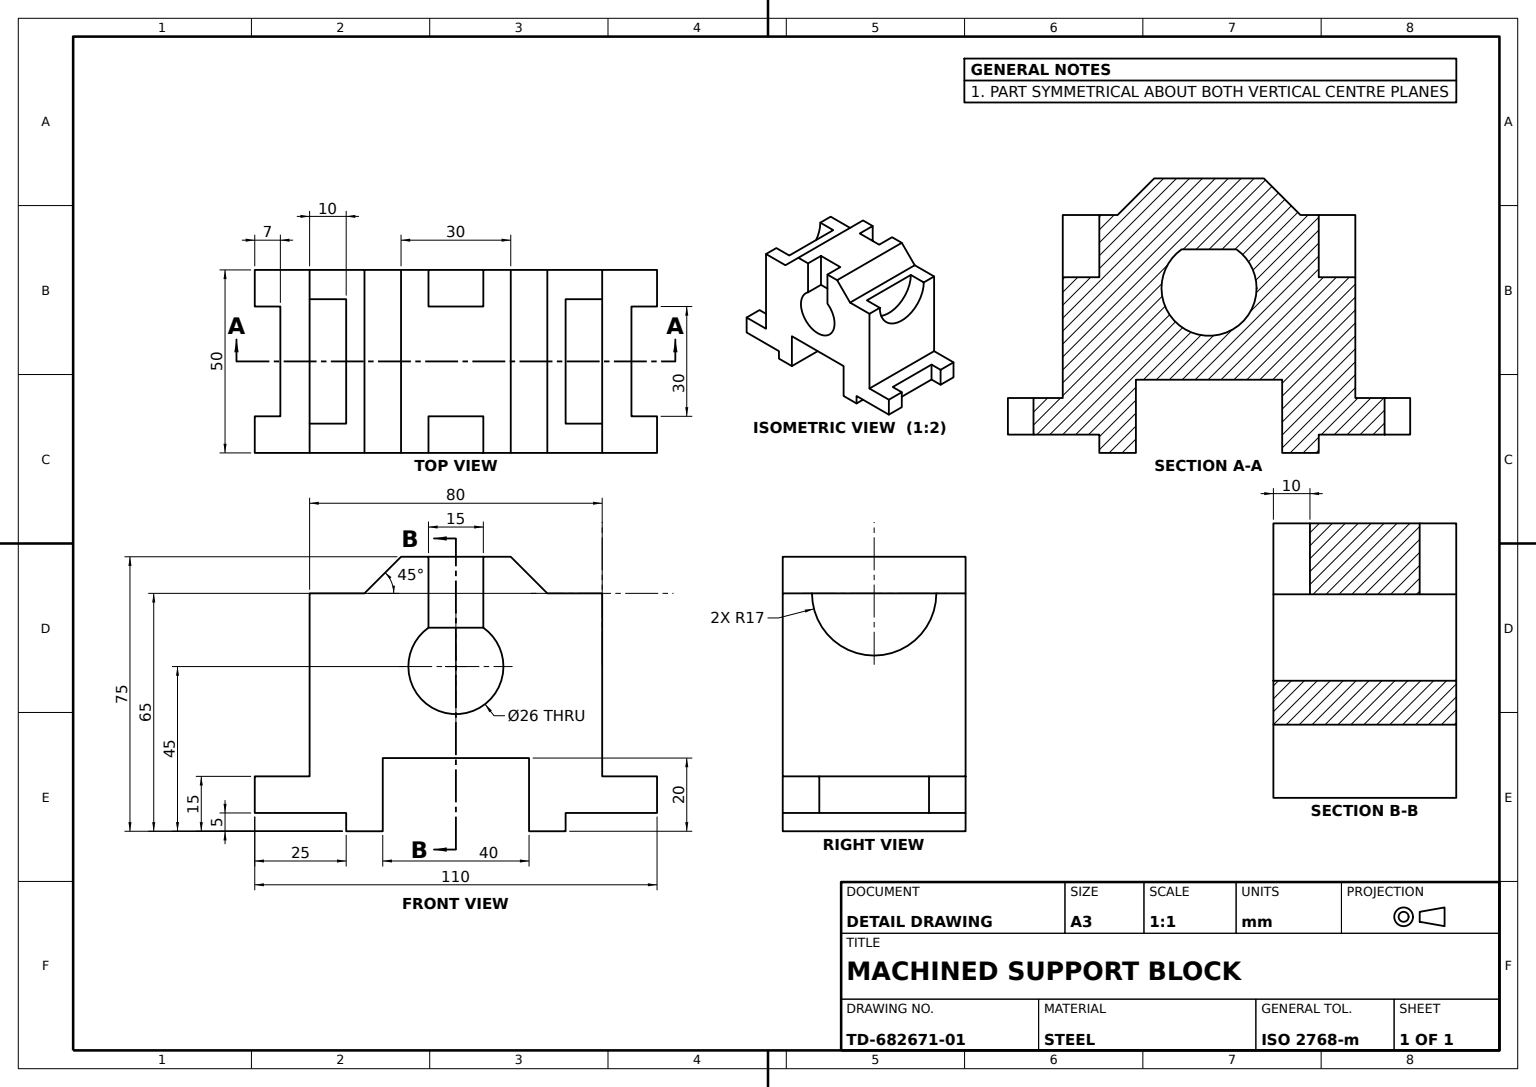
ISO-10303-21;
HEADER;
FILE_DESCRIPTION((''),'2;1');
FILE_NAME('','',(''),(''),'','','');
FILE_SCHEMA(('AUTOMOTIVE_DESIGN'));
ENDSEC;
DATA;
#1=APPLICATION_CONTEXT('');
#2=PRODUCT_CONTEXT('',#1,'mechanical');
#3=PRODUCT('','','',(#2));
#4=PRODUCT_DEFINITION_FORMATION('','',#3);
#5=PRODUCT_DEFINITION_CONTEXT('',#1,'design');
#6=PRODUCT_DEFINITION('','',#4,#5);
#7=PRODUCT_DEFINITION_SHAPE('','',#6);
#8=(LENGTH_UNIT()NAMED_UNIT(*)SI_UNIT(.MILLI.,.METRE.));
#9=(NAMED_UNIT(*)PLANE_ANGLE_UNIT()SI_UNIT($,.RADIAN.));
#10=(NAMED_UNIT(*)SI_UNIT($,.STERADIAN.)SOLID_ANGLE_UNIT());
#11=UNCERTAINTY_MEASURE_WITH_UNIT(LENGTH_MEASURE(1.E-05),#8,'distance_accuracy_value','');
#12=(GEOMETRIC_REPRESENTATION_CONTEXT(3)GLOBAL_UNCERTAINTY_ASSIGNED_CONTEXT((#11))GLOBAL_UNIT_ASSIGNED_CONTEXT((#8,#9,#10))REPRESENTATION_CONTEXT('',''));
#13=CARTESIAN_POINT('',(25.,0.,13.));
#14=VERTEX_POINT('',#13);
#15=CARTESIAN_POINT('',(-25.,0.,13.));
#16=VERTEX_POINT('',#15);
#17=DIRECTION('',(-1.,0.,0.));
#18=VECTOR('',#17,1000.);
#19=LINE('',#13,#18);
#20=EDGE_CURVE('',#14,#16,#19,.T.);
#21=ORIENTED_EDGE('',*,*,#20,.T.);
#22=CARTESIAN_POINT('',(-25.,10.61838,7.5));
#23=VERTEX_POINT('',#22);
#24=CARTESIAN_POINT('',(-25.,0.,0.));
#25=DIRECTION('',(0.,0.,-1.));
#26=AXIS2_PLACEMENT_3D('',#24,#17,#25);
#27=CIRCLE('',#26,13.);
#28=EDGE_CURVE('',#16,#23,#27,.T.);
#29=ORIENTED_EDGE('',*,*,#28,.T.);
#30=CARTESIAN_POINT('',(-15.,10.61838,7.5));
#31=VERTEX_POINT('',#30);
#32=CARTESIAN_POINT('',(25.,10.61838,7.5));
#33=LINE('',#32,#18);
#34=EDGE_CURVE('',#31,#23,#33,.T.);
#35=ORIENTED_EDGE('',*,*,#34,.F.);
#36=CARTESIAN_POINT('',(15.,10.61838,7.5));
#37=VERTEX_POINT('',#36);
#38=LINE('',#36,#18);
#39=EDGE_CURVE('',#37,#31,#38,.T.);
#40=ORIENTED_EDGE('',*,*,#39,.F.);
#41=VERTEX_POINT('',#32);
#42=EDGE_CURVE('',#41,#37,#33,.T.);
#43=ORIENTED_EDGE('',*,*,#42,.F.);
#44=CARTESIAN_POINT('',(25.,0.,0.));
#45=AXIS2_PLACEMENT_3D('',#44,#17,#25);
#46=CIRCLE('',#45,13.);
#47=EDGE_CURVE('',#14,#41,#46,.T.);
#48=ORIENTED_EDGE('',*,*,#47,.F.);
#49=EDGE_LOOP('',(#21,#29,#35,#40,#43,#48));
#50=FACE_OUTER_BOUND('',#49,.T.);
#51=DIRECTION('',(0.,0.,1.));
#52=AXIS2_PLACEMENT_3D('',#44,#17,#51);
#53=CYLINDRICAL_SURFACE('',#52,13.);
#54=ADVANCED_FACE('',(#50),#53,.F.);
#55=CARTESIAN_POINT('',(25.,-45.,-30.));
#56=VERTEX_POINT('',#55);
#57=CARTESIAN_POINT('',(25.,-40.,-30.));
#58=VERTEX_POINT('',#57);
#59=DIRECTION('',(0.,1.,0.));
#60=VECTOR('',#59,1000.);
#61=LINE('',#55,#60);
#62=EDGE_CURVE('',#56,#58,#61,.T.);
#63=ORIENTED_EDGE('',*,*,#62,.T.);
#64=CARTESIAN_POINT('',(25.,-40.,-55.));
#65=VERTEX_POINT('',#64);
#66=VECTOR('',#25,1000.);
#67=LINE('',#57,#66);
#68=EDGE_CURVE('',#58,#65,#67,.T.);
#69=ORIENTED_EDGE('',*,*,#68,.T.);
#70=CARTESIAN_POINT('',(25.,-30.,-55.));
#71=VERTEX_POINT('',#70);
#72=LINE('',#64,#60);
#73=EDGE_CURVE('',#65,#71,#72,.T.);
#74=ORIENTED_EDGE('',*,*,#73,.T.);
#75=CARTESIAN_POINT('',(25.,-30.,-40.));
#76=VERTEX_POINT('',#75);
#77=VECTOR('',#51,1000.);
#78=LINE('',#70,#77);
#79=EDGE_CURVE('',#71,#76,#78,.T.);
#80=ORIENTED_EDGE('',*,*,#79,.T.);
#81=CARTESIAN_POINT('',(25.,20.,-40.));
#82=VERTEX_POINT('',#81);
#83=LINE('',#75,#60);
#84=EDGE_CURVE('',#76,#82,#83,.T.);
#85=ORIENTED_EDGE('',*,*,#84,.T.);
#86=CARTESIAN_POINT('',(25.,20.,-25.));
#87=VERTEX_POINT('',#86);
#88=LINE('',#81,#77);
#89=EDGE_CURVE('',#82,#87,#88,.T.);
#90=ORIENTED_EDGE('',*,*,#89,.T.);
#91=CARTESIAN_POINT('',(25.,30.,-15.));
#92=VERTEX_POINT('',#91);
#93=DIRECTION('',(0.,0.707106781,0.707106781));
#94=VECTOR('',#93,1000.);
#95=LINE('',#86,#94);
#96=EDGE_CURVE('',#87,#92,#95,.T.);
#97=ORIENTED_EDGE('',*,*,#96,.T.);
#98=CARTESIAN_POINT('',(25.,30.,-7.5));
#99=VERTEX_POINT('',#98);
#100=LINE('',#91,#77);
#101=EDGE_CURVE('',#92,#99,#100,.T.);
#102=ORIENTED_EDGE('',*,*,#101,.T.);
#103=CARTESIAN_POINT('',(25.,10.61838,-7.5));
#104=VERTEX_POINT('',#103);
#105=DIRECTION('',(0.,-1.,0.));
#106=VECTOR('',#105,1000.);
#107=LINE('',#98,#106);
#108=EDGE_CURVE('',#99,#104,#107,.T.);
#109=ORIENTED_EDGE('',*,*,#108,.T.);
#110=CARTESIAN_POINT('',(25.,0.,-13.));
#111=VERTEX_POINT('',#110);
#112=EDGE_CURVE('',#104,#111,#46,.T.);
#113=ORIENTED_EDGE('',*,*,#112,.T.);
#114=EDGE_CURVE('',#111,#14,#46,.T.);
#115=ORIENTED_EDGE('',*,*,#114,.T.);
#116=ORIENTED_EDGE('',*,*,#47,.T.);
#117=CARTESIAN_POINT('',(25.,30.,7.5));
#118=VERTEX_POINT('',#117);
#119=LINE('',#117,#60);
#120=EDGE_CURVE('',#41,#118,#119,.T.);
#121=ORIENTED_EDGE('',*,*,#120,.T.);
#122=CARTESIAN_POINT('',(25.,30.,15.));
#123=VERTEX_POINT('',#122);
#124=LINE('',#122,#77);
#125=EDGE_CURVE('',#118,#123,#124,.T.);
#126=ORIENTED_EDGE('',*,*,#125,.T.);
#127=CARTESIAN_POINT('',(25.,20.,25.));
#128=VERTEX_POINT('',#127);
#129=DIRECTION('',(0.,-0.707106781,0.707106781));
#130=VECTOR('',#129,1000.);
#131=LINE('',#127,#130);
#132=EDGE_CURVE('',#123,#128,#131,.T.);
#133=ORIENTED_EDGE('',*,*,#132,.T.);
#134=CARTESIAN_POINT('',(25.,20.,40.));
#135=VERTEX_POINT('',#134);
#136=LINE('',#134,#77);
#137=EDGE_CURVE('',#128,#135,#136,.T.);
#138=ORIENTED_EDGE('',*,*,#137,.T.);
#139=CARTESIAN_POINT('',(25.,-30.,40.));
#140=VERTEX_POINT('',#139);
#141=LINE('',#139,#106);
#142=EDGE_CURVE('',#135,#140,#141,.T.);
#143=ORIENTED_EDGE('',*,*,#142,.T.);
#144=CARTESIAN_POINT('',(25.,-30.,55.));
#145=VERTEX_POINT('',#144);
#146=LINE('',#144,#77);
#147=EDGE_CURVE('',#140,#145,#146,.T.);
#148=ORIENTED_EDGE('',*,*,#147,.T.);
#149=CARTESIAN_POINT('',(25.,-40.,55.));
#150=VERTEX_POINT('',#149);
#151=LINE('',#149,#106);
#152=EDGE_CURVE('',#145,#150,#151,.T.);
#153=ORIENTED_EDGE('',*,*,#152,.T.);
#154=CARTESIAN_POINT('',(25.,-40.,30.));
#155=VERTEX_POINT('',#154);
#156=LINE('',#154,#66);
#157=EDGE_CURVE('',#150,#155,#156,.T.);
#158=ORIENTED_EDGE('',*,*,#157,.T.);
#159=CARTESIAN_POINT('',(25.,-45.,30.));
#160=VERTEX_POINT('',#159);
#161=LINE('',#159,#106);
#162=EDGE_CURVE('',#155,#160,#161,.T.);
#163=ORIENTED_EDGE('',*,*,#162,.T.);
#164=CARTESIAN_POINT('',(25.,-45.,20.));
#165=VERTEX_POINT('',#164);
#166=LINE('',#164,#66);
#167=EDGE_CURVE('',#160,#165,#166,.T.);
#168=ORIENTED_EDGE('',*,*,#167,.T.);
#169=CARTESIAN_POINT('',(25.,-25.,20.));
#170=VERTEX_POINT('',#169);
#171=LINE('',#169,#60);
#172=EDGE_CURVE('',#165,#170,#171,.T.);
#173=ORIENTED_EDGE('',*,*,#172,.T.);
#174=CARTESIAN_POINT('',(25.,-25.,-20.));
#175=VERTEX_POINT('',#174);
#176=LINE('',#169,#66);
#177=EDGE_CURVE('',#170,#175,#176,.T.);
#178=ORIENTED_EDGE('',*,*,#177,.T.);
#179=CARTESIAN_POINT('',(25.,-45.,-20.));
#180=VERTEX_POINT('',#179);
#181=LINE('',#174,#106);
#182=EDGE_CURVE('',#175,#180,#181,.T.);
#183=ORIENTED_EDGE('',*,*,#182,.T.);
#184=LINE('',#179,#66);
#185=EDGE_CURVE('',#180,#56,#184,.T.);
#186=ORIENTED_EDGE('',*,*,#185,.T.);
#187=EDGE_LOOP('',(#63,#69,#74,#80,#85,#90,#97,#102,#109,#113,#115,#116,#121,#126,#133,#138,#143,#148,#153,#158,#163,#168,#173,#178,#183,#186));
#188=FACE_OUTER_BOUND('',#187,.T.);
#189=DIRECTION('',(1.,0.,0.));
#190=AXIS2_PLACEMENT_3D('',#44,#189,#25);
#191=PLANE('',#190);
#192=ADVANCED_FACE('',(#188),#191,.T.);
#193=ORIENTED_EDGE('',*,*,#42,.T.);
#194=CARTESIAN_POINT('',(15.,30.,7.5));
#195=VERTEX_POINT('',#194);
#196=LINE('',#194,#106);
#197=EDGE_CURVE('',#195,#37,#196,.T.);
#198=ORIENTED_EDGE('',*,*,#197,.F.);
#199=LINE('',#117,#18);
#200=EDGE_CURVE('',#118,#195,#199,.T.);
#201=ORIENTED_EDGE('',*,*,#200,.F.);
#202=ORIENTED_EDGE('',*,*,#120,.F.);
#203=EDGE_LOOP('',(#193,#198,#201,#202));
#204=FACE_OUTER_BOUND('',#203,.T.);
#205=AXIS2_PLACEMENT_3D('',#117,#51,#105);
#206=PLANE('',#205);
#207=ADVANCED_FACE('',(#204),#206,.F.);
#208=ORIENTED_EDGE('',*,*,#108,.F.);
#209=CARTESIAN_POINT('',(15.,30.,-7.5));
#210=VERTEX_POINT('',#209);
#211=LINE('',#98,#18);
#212=EDGE_CURVE('',#99,#210,#211,.T.);
#213=ORIENTED_EDGE('',*,*,#212,.T.);
#214=CARTESIAN_POINT('',(15.,10.61838,-7.5));
#215=VERTEX_POINT('',#214);
#216=LINE('',#209,#60);
#217=EDGE_CURVE('',#215,#210,#216,.T.);
#218=ORIENTED_EDGE('',*,*,#217,.F.);
#219=LINE('',#103,#18);
#220=EDGE_CURVE('',#104,#215,#219,.T.);
#221=ORIENTED_EDGE('',*,*,#220,.F.);
#222=EDGE_LOOP('',(#208,#213,#218,#221));
#223=FACE_OUTER_BOUND('',#222,.T.);
#224=AXIS2_PLACEMENT_3D('',#98,#25,#59);
#225=PLANE('',#224);
#226=ADVANCED_FACE('',(#223),#225,.F.);
#227=CARTESIAN_POINT('',(-15.,30.,7.5));
#228=VERTEX_POINT('',#227);
#229=CARTESIAN_POINT('',(-25.,30.,7.5));
#230=VERTEX_POINT('',#229);
#231=EDGE_CURVE('',#228,#230,#199,.T.);
#232=ORIENTED_EDGE('',*,*,#231,.F.);
#233=LINE('',#227,#106);
#234=EDGE_CURVE('',#228,#31,#233,.T.);
#235=ORIENTED_EDGE('',*,*,#234,.T.);
#236=ORIENTED_EDGE('',*,*,#34,.T.);
#237=LINE('',#229,#60);
#238=EDGE_CURVE('',#23,#230,#237,.T.);
#239=ORIENTED_EDGE('',*,*,#238,.T.);
#240=EDGE_LOOP('',(#232,#235,#236,#239));
#241=FACE_OUTER_BOUND('',#240,.T.);
#242=ADVANCED_FACE('',(#241),#206,.F.);
#243=CARTESIAN_POINT('',(-15.,-30.,-55.));
#244=VERTEX_POINT('',#243);
#245=CARTESIAN_POINT('',(-25.,-30.,-55.));
#246=VERTEX_POINT('',#245);
#247=LINE('',#70,#18);
#248=EDGE_CURVE('',#244,#246,#247,.T.);
#249=ORIENTED_EDGE('',*,*,#248,.T.);
#250=CARTESIAN_POINT('',(-25.,-30.,-40.));
#251=VERTEX_POINT('',#250);
#252=LINE('',#245,#77);
#253=EDGE_CURVE('',#246,#251,#252,.T.);
#254=ORIENTED_EDGE('',*,*,#253,.T.);
#255=LINE('',#75,#18);
#256=EDGE_CURVE('',#76,#251,#255,.T.);
#257=ORIENTED_EDGE('',*,*,#256,.F.);
#258=ORIENTED_EDGE('',*,*,#79,.F.);
#259=CARTESIAN_POINT('',(15.,-30.,-55.));
#260=VERTEX_POINT('',#259);
#261=EDGE_CURVE('',#71,#260,#247,.T.);
#262=ORIENTED_EDGE('',*,*,#261,.T.);
#263=CARTESIAN_POINT('',(15.,-30.,-48.));
#264=VERTEX_POINT('',#263);
#265=LINE('',#263,#66);
#266=EDGE_CURVE('',#264,#260,#265,.T.);
#267=ORIENTED_EDGE('',*,*,#266,.F.);
#268=CARTESIAN_POINT('',(-15.,-30.,-48.));
#269=VERTEX_POINT('',#268);
#270=LINE('',#268,#18);
#271=EDGE_CURVE('',#264,#269,#270,.T.);
#272=ORIENTED_EDGE('',*,*,#271,.T.);
#273=LINE('',#268,#66);
#274=EDGE_CURVE('',#269,#244,#273,.T.);
#275=ORIENTED_EDGE('',*,*,#274,.T.);
#276=EDGE_LOOP('',(#249,#254,#257,#258,#262,#267,#272,#275));
#277=FACE_OUTER_BOUND('',#276,.T.);
#278=AXIS2_PLACEMENT_3D('',#70,#105,#25);
#279=PLANE('',#278);
#280=ADVANCED_FACE('',(#277),#279,.F.);
#281=CARTESIAN_POINT('',(-15.,-40.,-48.));
#282=VERTEX_POINT('',#281);
#283=CARTESIAN_POINT('',(-15.,-40.,-55.));
#284=VERTEX_POINT('',#283);
#285=LINE('',#281,#66);
#286=EDGE_CURVE('',#282,#284,#285,.T.);
#287=ORIENTED_EDGE('',*,*,#286,.T.);
#288=LINE('',#243,#106);
#289=EDGE_CURVE('',#244,#284,#288,.T.);
#290=ORIENTED_EDGE('',*,*,#289,.F.);
#291=ORIENTED_EDGE('',*,*,#274,.F.);
#292=LINE('',#268,#106);
#293=EDGE_CURVE('',#269,#282,#292,.T.);
#294=ORIENTED_EDGE('',*,*,#293,.T.);
#295=EDGE_LOOP('',(#287,#290,#291,#294));
#296=FACE_OUTER_BOUND('',#295,.T.);
#297=AXIS2_PLACEMENT_3D('',#268,#189,#59);
#298=PLANE('',#297);
#299=ADVANCED_FACE('',(#296),#298,.T.);
#300=CARTESIAN_POINT('',(-17.,20.,-30.));
#301=VERTEX_POINT('',#300);
#302=CARTESIAN_POINT('',(-17.,20.,-40.));
#303=VERTEX_POINT('',#302);
#304=LINE('',#300,#66);
#305=EDGE_CURVE('',#301,#303,#304,.T.);
#306=ORIENTED_EDGE('',*,*,#305,.T.);
#307=CARTESIAN_POINT('',(-25.,20.,-40.));
#308=VERTEX_POINT('',#307);
#309=LINE('',#81,#18);
#310=EDGE_CURVE('',#303,#308,#309,.T.);
#311=ORIENTED_EDGE('',*,*,#310,.T.);
#312=CARTESIAN_POINT('',(-25.,20.,-25.));
#313=VERTEX_POINT('',#312);
#314=LINE('',#307,#77);
#315=EDGE_CURVE('',#308,#313,#314,.T.);
#316=ORIENTED_EDGE('',*,*,#315,.T.);
#317=LINE('',#86,#18);
#318=EDGE_CURVE('',#87,#313,#317,.T.);
#319=ORIENTED_EDGE('',*,*,#318,.F.);
#320=ORIENTED_EDGE('',*,*,#89,.F.);
#321=CARTESIAN_POINT('',(17.,20.,-40.));
#322=VERTEX_POINT('',#321);
#323=EDGE_CURVE('',#82,#322,#309,.T.);
#324=ORIENTED_EDGE('',*,*,#323,.T.);
#325=CARTESIAN_POINT('',(17.,20.,-30.));
#326=VERTEX_POINT('',#325);
#327=LINE('',#325,#66);
#328=EDGE_CURVE('',#326,#322,#327,.T.);
#329=ORIENTED_EDGE('',*,*,#328,.F.);
#330=LINE('',#300,#18);
#331=EDGE_CURVE('',#326,#301,#330,.T.);
#332=ORIENTED_EDGE('',*,*,#331,.T.);
#333=EDGE_LOOP('',(#306,#311,#316,#319,#320,#324,#329,#332));
#334=FACE_OUTER_BOUND('',#333,.T.);
#335=AXIS2_PLACEMENT_3D('',#81,#105,#25);
#336=PLANE('',#335);
#337=ADVANCED_FACE('',(#334),#336,.F.);
#338=CARTESIAN_POINT('',(15.,-40.,-55.));
#339=VERTEX_POINT('',#338);
#340=LINE('',#259,#60);
#341=EDGE_CURVE('',#339,#260,#340,.T.);
#342=ORIENTED_EDGE('',*,*,#341,.T.);
#343=ORIENTED_EDGE('',*,*,#261,.F.);
#344=ORIENTED_EDGE('',*,*,#73,.F.);
#345=LINE('',#64,#18);
#346=EDGE_CURVE('',#65,#339,#345,.T.);
#347=ORIENTED_EDGE('',*,*,#346,.T.);
#348=EDGE_LOOP('',(#342,#343,#344,#347));
#349=FACE_OUTER_BOUND('',#348,.T.);
#350=AXIS2_PLACEMENT_3D('',#64,#51,#189);
#351=PLANE('',#350);
#352=ADVANCED_FACE('',(#349),#351,.F.);
#353=CARTESIAN_POINT('',(-25.,-45.,-20.));
#354=VERTEX_POINT('',#353);
#355=LINE('',#179,#18);
#356=EDGE_CURVE('',#180,#354,#355,.T.);
#357=ORIENTED_EDGE('',*,*,#356,.T.);
#358=CARTESIAN_POINT('',(-25.,-45.,-30.));
#359=VERTEX_POINT('',#358);
#360=LINE('',#353,#66);
#361=EDGE_CURVE('',#354,#359,#360,.T.);
#362=ORIENTED_EDGE('',*,*,#361,.T.);
#363=LINE('',#55,#18);
#364=EDGE_CURVE('',#56,#359,#363,.T.);
#365=ORIENTED_EDGE('',*,*,#364,.F.);
#366=ORIENTED_EDGE('',*,*,#185,.F.);
#367=EDGE_LOOP('',(#357,#362,#365,#366));
#368=FACE_OUTER_BOUND('',#367,.T.);
#369=AXIS2_PLACEMENT_3D('',#179,#59,#51);
#370=PLANE('',#369);
#371=ADVANCED_FACE('',(#368),#370,.F.);
#372=CARTESIAN_POINT('',(-15.,-40.,48.));
#373=VERTEX_POINT('',#372);
#374=CARTESIAN_POINT('',(15.,-40.,48.));
#375=VERTEX_POINT('',#374);
#376=VECTOR('',#189,1000.);
#377=LINE('',#372,#376);
#378=EDGE_CURVE('',#373,#375,#377,.T.);
#379=ORIENTED_EDGE('',*,*,#378,.F.);
#380=CARTESIAN_POINT('',(-15.,-40.,55.));
#381=VERTEX_POINT('',#380);
#382=LINE('',#372,#77);
#383=EDGE_CURVE('',#373,#381,#382,.T.);
#384=ORIENTED_EDGE('',*,*,#383,.T.);
#385=CARTESIAN_POINT('',(-25.,-40.,55.));
#386=VERTEX_POINT('',#385);
#387=LINE('',#149,#18);
#388=EDGE_CURVE('',#381,#386,#387,.T.);
#389=ORIENTED_EDGE('',*,*,#388,.T.);
#390=CARTESIAN_POINT('',(-25.,-40.,30.));
#391=VERTEX_POINT('',#390);
#392=LINE('',#390,#66);
#393=EDGE_CURVE('',#386,#391,#392,.T.);
#394=ORIENTED_EDGE('',*,*,#393,.T.);
#395=LINE('',#154,#18);
#396=EDGE_CURVE('',#155,#391,#395,.T.);
#397=ORIENTED_EDGE('',*,*,#396,.F.);
#398=ORIENTED_EDGE('',*,*,#157,.F.);
#399=CARTESIAN_POINT('',(15.,-40.,55.));
#400=VERTEX_POINT('',#399);
#401=EDGE_CURVE('',#150,#400,#387,.T.);
#402=ORIENTED_EDGE('',*,*,#401,.T.);
#403=LINE('',#374,#77);
#404=EDGE_CURVE('',#375,#400,#403,.T.);
#405=ORIENTED_EDGE('',*,*,#404,.F.);
#406=EDGE_LOOP('',(#379,#384,#389,#394,#397,#398,#402,#405));
#407=FACE_OUTER_BOUND('',#406,.T.);
#408=AXIS2_PLACEMENT_3D('',#154,#59,#51);
#409=PLANE('',#408);
#410=ADVANCED_FACE('',(#407),#409,.F.);
#411=ORIENTED_EDGE('',*,*,#346,.F.);
#412=ORIENTED_EDGE('',*,*,#68,.F.);
#413=CARTESIAN_POINT('',(-25.,-40.,-30.));
#414=VERTEX_POINT('',#413);
#415=LINE('',#57,#18);
#416=EDGE_CURVE('',#58,#414,#415,.T.);
#417=ORIENTED_EDGE('',*,*,#416,.T.);
#418=CARTESIAN_POINT('',(-25.,-40.,-55.));
#419=VERTEX_POINT('',#418);
#420=LINE('',#413,#66);
#421=EDGE_CURVE('',#414,#419,#420,.T.);
#422=ORIENTED_EDGE('',*,*,#421,.T.);
#423=EDGE_CURVE('',#284,#419,#345,.T.);
#424=ORIENTED_EDGE('',*,*,#423,.F.);
#425=ORIENTED_EDGE('',*,*,#286,.F.);
#426=CARTESIAN_POINT('',(15.,-40.,-48.));
#427=VERTEX_POINT('',#426);
#428=LINE('',#281,#376);
#429=EDGE_CURVE('',#282,#427,#428,.T.);
#430=ORIENTED_EDGE('',*,*,#429,.T.);
#431=LINE('',#426,#66);
#432=EDGE_CURVE('',#427,#339,#431,.T.);
#433=ORIENTED_EDGE('',*,*,#432,.T.);
#434=EDGE_LOOP('',(#411,#412,#417,#422,#424,#425,#430,#433));
#435=FACE_OUTER_BOUND('',#434,.T.);
#436=AXIS2_PLACEMENT_3D('',#57,#59,#51);
#437=PLANE('',#436);
#438=ADVANCED_FACE('',(#435),#437,.F.);
#439=ORIENTED_EDGE('',*,*,#396,.T.);
#440=CARTESIAN_POINT('',(-25.,-45.,30.));
#441=VERTEX_POINT('',#440);
#442=LINE('',#440,#106);
#443=EDGE_CURVE('',#391,#441,#442,.T.);
#444=ORIENTED_EDGE('',*,*,#443,.T.);
#445=LINE('',#159,#18);
#446=EDGE_CURVE('',#160,#441,#445,.T.);
#447=ORIENTED_EDGE('',*,*,#446,.F.);
#448=ORIENTED_EDGE('',*,*,#162,.F.);
#449=EDGE_LOOP('',(#439,#444,#447,#448));
#450=FACE_OUTER_BOUND('',#449,.T.);
#451=AXIS2_PLACEMENT_3D('',#159,#25,#17);
#452=PLANE('',#451);
#453=ADVANCED_FACE('',(#450),#452,.F.);
#454=CARTESIAN_POINT('',(-25.,-30.,55.));
#455=VERTEX_POINT('',#454);
#456=LINE('',#385,#106);
#457=EDGE_CURVE('',#455,#386,#456,.T.);
#458=ORIENTED_EDGE('',*,*,#457,.T.);
#459=ORIENTED_EDGE('',*,*,#388,.F.);
#460=CARTESIAN_POINT('',(-15.,-30.,55.));
#461=VERTEX_POINT('',#460);
#462=LINE('',#460,#106);
#463=EDGE_CURVE('',#461,#381,#462,.T.);
#464=ORIENTED_EDGE('',*,*,#463,.F.);
#465=LINE('',#144,#18);
#466=EDGE_CURVE('',#461,#455,#465,.T.);
#467=ORIENTED_EDGE('',*,*,#466,.T.);
#468=EDGE_LOOP('',(#458,#459,#464,#467));
#469=FACE_OUTER_BOUND('',#468,.T.);
#470=AXIS2_PLACEMENT_3D('',#149,#25,#17);
#471=PLANE('',#470);
#472=ADVANCED_FACE('',(#469),#471,.F.);
#473=CARTESIAN_POINT('',(-15.,-30.,48.));
#474=VERTEX_POINT('',#473);
#475=LINE('',#473,#77);
#476=EDGE_CURVE('',#474,#461,#475,.T.);
#477=ORIENTED_EDGE('',*,*,#476,.T.);
#478=ORIENTED_EDGE('',*,*,#463,.T.);
#479=ORIENTED_EDGE('',*,*,#383,.F.);
#480=LINE('',#473,#106);
#481=EDGE_CURVE('',#474,#373,#480,.T.);
#482=ORIENTED_EDGE('',*,*,#481,.F.);
#483=EDGE_LOOP('',(#477,#478,#479,#482));
#484=FACE_OUTER_BOUND('',#483,.T.);
#485=AXIS2_PLACEMENT_3D('',#473,#17,#105);
#486=PLANE('',#485);
#487=ADVANCED_FACE('',(#484),#486,.F.);
#488=CARTESIAN_POINT('',(-25.,-25.,20.));
#489=VERTEX_POINT('',#488);
#490=LINE('',#169,#18);
#491=EDGE_CURVE('',#170,#489,#490,.T.);
#492=ORIENTED_EDGE('',*,*,#491,.T.);
#493=CARTESIAN_POINT('',(-25.,-25.,-20.));
#494=VERTEX_POINT('',#493);
#495=LINE('',#488,#66);
#496=EDGE_CURVE('',#489,#494,#495,.T.);
#497=ORIENTED_EDGE('',*,*,#496,.T.);
#498=LINE('',#174,#18);
#499=EDGE_CURVE('',#175,#494,#498,.T.);
#500=ORIENTED_EDGE('',*,*,#499,.F.);
#501=ORIENTED_EDGE('',*,*,#177,.F.);
#502=EDGE_LOOP('',(#492,#497,#500,#501));
#503=FACE_OUTER_BOUND('',#502,.T.);
#504=AXIS2_PLACEMENT_3D('',#169,#59,#51);
#505=PLANE('',#504);
#506=ADVANCED_FACE('',(#503),#505,.F.);
#507=ORIENTED_EDGE('',*,*,#271,.F.);
#508=LINE('',#263,#60);
#509=EDGE_CURVE('',#427,#264,#508,.T.);
#510=ORIENTED_EDGE('',*,*,#509,.F.);
#511=ORIENTED_EDGE('',*,*,#429,.F.);
#512=ORIENTED_EDGE('',*,*,#293,.F.);
#513=EDGE_LOOP('',(#507,#510,#511,#512));
#514=FACE_OUTER_BOUND('',#513,.T.);
#515=CARTESIAN_POINT('',(0.,0.,-48.));
#516=AXIS2_PLACEMENT_3D('',#515,#25,#189);
#517=PLANE('',#516);
#518=ADVANCED_FACE('',(#514),#517,.T.);
#519=ORIENTED_EDGE('',*,*,#84,.F.);
#520=ORIENTED_EDGE('',*,*,#256,.T.);
#521=LINE('',#250,#60);
#522=EDGE_CURVE('',#251,#308,#521,.T.);
#523=ORIENTED_EDGE('',*,*,#522,.T.);
#524=ORIENTED_EDGE('',*,*,#310,.F.);
#525=CARTESIAN_POINT('',(0.,20.,-40.));
#526=AXIS2_PLACEMENT_3D('',#525,#51,#189);
#527=CIRCLE('',#526,17.);
#528=EDGE_CURVE('',#303,#322,#527,.T.);
#529=ORIENTED_EDGE('',*,*,#528,.T.);
#530=ORIENTED_EDGE('',*,*,#323,.F.);
#531=EDGE_LOOP('',(#519,#520,#523,#524,#529,#530));
#532=FACE_OUTER_BOUND('',#531,.T.);
#533=AXIS2_PLACEMENT_3D('',#75,#51,#189);
#534=PLANE('',#533);
#535=ADVANCED_FACE('',(#532),#534,.F.);
#536=CARTESIAN_POINT('',(-25.,-45.,20.));
#537=VERTEX_POINT('',#536);
#538=LINE('',#164,#18);
#539=EDGE_CURVE('',#165,#537,#538,.T.);
#540=ORIENTED_EDGE('',*,*,#539,.T.);
#541=LINE('',#488,#60);
#542=EDGE_CURVE('',#537,#489,#541,.T.);
#543=ORIENTED_EDGE('',*,*,#542,.T.);
#544=ORIENTED_EDGE('',*,*,#491,.F.);
#545=ORIENTED_EDGE('',*,*,#172,.F.);
#546=EDGE_LOOP('',(#540,#543,#544,#545));
#547=FACE_OUTER_BOUND('',#546,.T.);
#548=AXIS2_PLACEMENT_3D('',#169,#51,#105);
#549=PLANE('',#548);
#550=ADVANCED_FACE('',(#547),#549,.F.);
#551=ORIENTED_EDGE('',*,*,#378,.T.);
#552=CARTESIAN_POINT('',(15.,-30.,48.));
#553=VERTEX_POINT('',#552);
#554=LINE('',#552,#60);
#555=EDGE_CURVE('',#375,#553,#554,.T.);
#556=ORIENTED_EDGE('',*,*,#555,.T.);
#557=LINE('',#473,#18);
#558=EDGE_CURVE('',#553,#474,#557,.T.);
#559=ORIENTED_EDGE('',*,*,#558,.T.);
#560=ORIENTED_EDGE('',*,*,#481,.T.);
#561=EDGE_LOOP('',(#551,#556,#559,#560));
#562=FACE_OUTER_BOUND('',#561,.T.);
#563=CARTESIAN_POINT('',(0.,0.,48.));
#564=AXIS2_PLACEMENT_3D('',#563,#51,#189);
#565=PLANE('',#564);
#566=ADVANCED_FACE('',(#562),#565,.T.);
#567=CARTESIAN_POINT('',(-17.,20.,40.));
#568=VERTEX_POINT('',#567);
#569=CARTESIAN_POINT('',(-25.,20.,40.));
#570=VERTEX_POINT('',#569);
#571=LINE('',#134,#18);
#572=EDGE_CURVE('',#568,#570,#571,.T.);
#573=ORIENTED_EDGE('',*,*,#572,.F.);
#574=CARTESIAN_POINT('',(-17.,20.,30.));
#575=VERTEX_POINT('',#574);
#576=LINE('',#574,#77);
#577=EDGE_CURVE('',#575,#568,#576,.T.);
#578=ORIENTED_EDGE('',*,*,#577,.F.);
#579=CARTESIAN_POINT('',(17.,20.,30.));
#580=VERTEX_POINT('',#579);
#581=LINE('',#574,#18);
#582=EDGE_CURVE('',#580,#575,#581,.T.);
#583=ORIENTED_EDGE('',*,*,#582,.F.);
#584=CARTESIAN_POINT('',(17.,20.,40.));
#585=VERTEX_POINT('',#584);
#586=LINE('',#579,#77);
#587=EDGE_CURVE('',#580,#585,#586,.T.);
#588=ORIENTED_EDGE('',*,*,#587,.T.);
#589=EDGE_CURVE('',#135,#585,#571,.T.);
#590=ORIENTED_EDGE('',*,*,#589,.F.);
#591=ORIENTED_EDGE('',*,*,#137,.F.);
#592=CARTESIAN_POINT('',(-25.,20.,25.));
#593=VERTEX_POINT('',#592);
#594=LINE('',#127,#18);
#595=EDGE_CURVE('',#128,#593,#594,.T.);
#596=ORIENTED_EDGE('',*,*,#595,.T.);
#597=LINE('',#569,#77);
#598=EDGE_CURVE('',#593,#570,#597,.T.);
#599=ORIENTED_EDGE('',*,*,#598,.T.);
#600=EDGE_LOOP('',(#573,#578,#583,#588,#590,#591,#596,#599));
#601=FACE_OUTER_BOUND('',#600,.T.);
#602=AXIS2_PLACEMENT_3D('',#134,#105,#25);
#603=PLANE('',#602);
#604=ADVANCED_FACE('',(#601),#603,.F.);
#605=ORIENTED_EDGE('',*,*,#152,.F.);
#606=CARTESIAN_POINT('',(15.,-30.,55.));
#607=VERTEX_POINT('',#606);
#608=EDGE_CURVE('',#145,#607,#465,.T.);
#609=ORIENTED_EDGE('',*,*,#608,.T.);
#610=LINE('',#606,#60);
#611=EDGE_CURVE('',#400,#607,#610,.T.);
#612=ORIENTED_EDGE('',*,*,#611,.F.);
#613=ORIENTED_EDGE('',*,*,#401,.F.);
#614=EDGE_LOOP('',(#605,#609,#612,#613));
#615=FACE_OUTER_BOUND('',#614,.T.);
#616=ADVANCED_FACE('',(#615),#471,.F.);
#617=ORIENTED_EDGE('',*,*,#423,.T.);
#618=LINE('',#418,#60);
#619=EDGE_CURVE('',#419,#246,#618,.T.);
#620=ORIENTED_EDGE('',*,*,#619,.T.);
#621=ORIENTED_EDGE('',*,*,#248,.F.);
#622=ORIENTED_EDGE('',*,*,#289,.T.);
#623=EDGE_LOOP('',(#617,#620,#621,#622));
#624=FACE_OUTER_BOUND('',#623,.T.);
#625=ADVANCED_FACE('',(#624),#351,.F.);
#626=CARTESIAN_POINT('',(-25.,30.,-15.));
#627=VERTEX_POINT('',#626);
#628=LINE('',#312,#94);
#629=EDGE_CURVE('',#313,#627,#628,.T.);
#630=ORIENTED_EDGE('',*,*,#629,.T.);
#631=LINE('',#91,#18);
#632=EDGE_CURVE('',#92,#627,#631,.T.);
#633=ORIENTED_EDGE('',*,*,#632,.F.);
#634=ORIENTED_EDGE('',*,*,#96,.F.);
#635=ORIENTED_EDGE('',*,*,#318,.T.);
#636=EDGE_LOOP('',(#630,#633,#634,#635));
#637=FACE_OUTER_BOUND('',#636,.T.);
#638=DIRECTION('',(0.,-0.707106781,-0.707106781));
#639=AXIS2_PLACEMENT_3D('',#86,#129,#638);
#640=PLANE('',#639);
#641=ADVANCED_FACE('',(#637),#640,.F.);
#642=CARTESIAN_POINT('',(-25.,30.,-7.5));
#643=VERTEX_POINT('',#642);
#644=CARTESIAN_POINT('',(-25.,10.61838,-7.5));
#645=VERTEX_POINT('',#644);
#646=LINE('',#642,#106);
#647=EDGE_CURVE('',#643,#645,#646,.T.);
#648=ORIENTED_EDGE('',*,*,#647,.T.);
#649=CARTESIAN_POINT('',(-15.,10.61838,-7.5));
#650=VERTEX_POINT('',#649);
#651=EDGE_CURVE('',#650,#645,#219,.T.);
#652=ORIENTED_EDGE('',*,*,#651,.F.);
#653=CARTESIAN_POINT('',(-15.,30.,-7.5));
#654=VERTEX_POINT('',#653);
#655=LINE('',#653,#60);
#656=EDGE_CURVE('',#650,#654,#655,.T.);
#657=ORIENTED_EDGE('',*,*,#656,.T.);
#658=EDGE_CURVE('',#654,#643,#211,.T.);
#659=ORIENTED_EDGE('',*,*,#658,.T.);
#660=EDGE_LOOP('',(#648,#652,#657,#659));
#661=FACE_OUTER_BOUND('',#660,.T.);
#662=ADVANCED_FACE('',(#661),#225,.F.);
#663=CARTESIAN_POINT('',(-25.,0.,-13.));
#664=VERTEX_POINT('',#663);
#665=LINE('',#110,#18);
#666=EDGE_CURVE('',#111,#664,#665,.T.);
#667=ORIENTED_EDGE('',*,*,#666,.T.);
#668=EDGE_CURVE('',#664,#16,#27,.T.);
#669=ORIENTED_EDGE('',*,*,#668,.T.);
#670=ORIENTED_EDGE('',*,*,#20,.F.);
#671=ORIENTED_EDGE('',*,*,#114,.F.);
#672=EDGE_LOOP('',(#667,#669,#670,#671));
#673=FACE_OUTER_BOUND('',#672,.T.);
#674=ADVANCED_FACE('',(#673),#53,.F.);
#675=ORIENTED_EDGE('',*,*,#572,.T.);
#676=CARTESIAN_POINT('',(-25.,-30.,40.));
#677=VERTEX_POINT('',#676);
#678=LINE('',#676,#106);
#679=EDGE_CURVE('',#570,#677,#678,.T.);
#680=ORIENTED_EDGE('',*,*,#679,.T.);
#681=LINE('',#139,#18);
#682=EDGE_CURVE('',#140,#677,#681,.T.);
#683=ORIENTED_EDGE('',*,*,#682,.F.);
#684=ORIENTED_EDGE('',*,*,#142,.F.);
#685=ORIENTED_EDGE('',*,*,#589,.T.);
#686=CARTESIAN_POINT('',(0.,20.,40.));
#687=AXIS2_PLACEMENT_3D('',#686,#51,#189);
#688=CIRCLE('',#687,17.);
#689=EDGE_CURVE('',#568,#585,#688,.T.);
#690=ORIENTED_EDGE('',*,*,#689,.F.);
#691=EDGE_LOOP('',(#675,#680,#683,#684,#685,#690));
#692=FACE_OUTER_BOUND('',#691,.T.);
#693=AXIS2_PLACEMENT_3D('',#139,#25,#17);
#694=PLANE('',#693);
#695=ADVANCED_FACE('',(#692),#694,.F.);
#696=ORIENTED_EDGE('',*,*,#132,.F.);
#697=CARTESIAN_POINT('',(-25.,30.,15.));
#698=VERTEX_POINT('',#697);
#699=LINE('',#122,#18);
#700=EDGE_CURVE('',#123,#698,#699,.T.);
#701=ORIENTED_EDGE('',*,*,#700,.T.);
#702=LINE('',#592,#130);
#703=EDGE_CURVE('',#698,#593,#702,.T.);
#704=ORIENTED_EDGE('',*,*,#703,.T.);
#705=ORIENTED_EDGE('',*,*,#595,.F.);
#706=EDGE_LOOP('',(#696,#701,#704,#705));
#707=FACE_OUTER_BOUND('',#706,.T.);
#708=DIRECTION('',(0.,0.707106781,-0.707106781));
#709=AXIS2_PLACEMENT_3D('',#127,#638,#708);
#710=PLANE('',#709);
#711=ADVANCED_FACE('',(#707),#710,.F.);
#712=LINE('',#36,#66);
#713=EDGE_CURVE('',#37,#215,#712,.T.);
#714=ORIENTED_EDGE('',*,*,#713,.F.);
#715=ORIENTED_EDGE('',*,*,#39,.T.);
#716=LINE('',#30,#66);
#717=EDGE_CURVE('',#31,#650,#716,.T.);
#718=ORIENTED_EDGE('',*,*,#717,.T.);
#719=LINE('',#214,#18);
#720=EDGE_CURVE('',#215,#650,#719,.T.);
#721=ORIENTED_EDGE('',*,*,#720,.F.);
#722=EDGE_LOOP('',(#714,#715,#718,#721));
#723=FACE_OUTER_BOUND('',#722,.T.);
#724=AXIS2_PLACEMENT_3D('',#36,#59,#51);
#725=PLANE('',#724);
#726=ADVANCED_FACE('',(#723),#725,.F.);
#727=ORIENTED_EDGE('',*,*,#266,.T.);
#728=ORIENTED_EDGE('',*,*,#341,.F.);
#729=ORIENTED_EDGE('',*,*,#432,.F.);
#730=ORIENTED_EDGE('',*,*,#509,.T.);
#731=EDGE_LOOP('',(#727,#728,#729,#730));
#732=FACE_OUTER_BOUND('',#731,.T.);
#733=AXIS2_PLACEMENT_3D('',#263,#17,#105);
#734=PLANE('',#733);
#735=ADVANCED_FACE('',(#732),#734,.T.);
#736=LINE('',#536,#66);
#737=EDGE_CURVE('',#441,#537,#736,.T.);
#738=ORIENTED_EDGE('',*,*,#737,.T.);
#739=ORIENTED_EDGE('',*,*,#539,.F.);
#740=ORIENTED_EDGE('',*,*,#167,.F.);
#741=ORIENTED_EDGE('',*,*,#446,.T.);
#742=EDGE_LOOP('',(#738,#739,#740,#741));
#743=FACE_OUTER_BOUND('',#742,.T.);
#744=AXIS2_PLACEMENT_3D('',#164,#59,#51);
#745=PLANE('',#744);
#746=ADVANCED_FACE('',(#743),#745,.F.);
#747=ORIENTED_EDGE('',*,*,#234,.F.);
#748=LINE('',#227,#77);
#749=EDGE_CURVE('',#654,#228,#748,.T.);
#750=ORIENTED_EDGE('',*,*,#749,.F.);
#751=ORIENTED_EDGE('',*,*,#656,.F.);
#752=ORIENTED_EDGE('',*,*,#717,.F.);
#753=EDGE_LOOP('',(#747,#750,#751,#752));
#754=FACE_OUTER_BOUND('',#753,.T.);
#755=CARTESIAN_POINT('',(-15.,0.,0.));
#756=AXIS2_PLACEMENT_3D('',#755,#189,#25);
#757=PLANE('',#756);
#758=ADVANCED_FACE('',(#754),#757,.F.);
#759=ORIENTED_EDGE('',*,*,#147,.F.);
#760=ORIENTED_EDGE('',*,*,#682,.T.);
#761=LINE('',#454,#77);
#762=EDGE_CURVE('',#677,#455,#761,.T.);
#763=ORIENTED_EDGE('',*,*,#762,.T.);
#764=ORIENTED_EDGE('',*,*,#466,.F.);
#765=ORIENTED_EDGE('',*,*,#476,.F.);
#766=ORIENTED_EDGE('',*,*,#558,.F.);
#767=LINE('',#552,#77);
#768=EDGE_CURVE('',#553,#607,#767,.T.);
#769=ORIENTED_EDGE('',*,*,#768,.T.);
#770=ORIENTED_EDGE('',*,*,#608,.F.);
#771=EDGE_LOOP('',(#759,#760,#763,#764,#765,#766,#769,#770));
#772=FACE_OUTER_BOUND('',#771,.T.);
#773=AXIS2_PLACEMENT_3D('',#144,#105,#25);
#774=PLANE('',#773);
#775=ADVANCED_FACE('',(#772),#774,.F.);
#776=CARTESIAN_POINT('',(0.,20.,30.));
#777=AXIS2_PLACEMENT_3D('',#776,#51,#189);
#778=CIRCLE('',#777,17.);
#779=EDGE_CURVE('',#575,#580,#778,.T.);
#780=ORIENTED_EDGE('',*,*,#779,.F.);
#781=ORIENTED_EDGE('',*,*,#577,.T.);
#782=ORIENTED_EDGE('',*,*,#689,.T.);
#783=ORIENTED_EDGE('',*,*,#587,.F.);
#784=EDGE_LOOP('',(#780,#781,#782,#783));
#785=FACE_OUTER_BOUND('',#784,.T.);
#786=CYLINDRICAL_SURFACE('',#777,17.);
#787=ADVANCED_FACE('',(#785),#786,.F.);
#788=ORIENTED_EDGE('',*,*,#555,.F.);
#789=ORIENTED_EDGE('',*,*,#404,.T.);
#790=ORIENTED_EDGE('',*,*,#611,.T.);
#791=ORIENTED_EDGE('',*,*,#768,.F.);
#792=EDGE_LOOP('',(#788,#789,#790,#791));
#793=FACE_OUTER_BOUND('',#792,.T.);
#794=AXIS2_PLACEMENT_3D('',#552,#189,#59);
#795=PLANE('',#794);
#796=ADVANCED_FACE('',(#793),#795,.F.);
#797=ORIENTED_EDGE('',*,*,#305,.F.);
#798=CARTESIAN_POINT('',(0.,20.,-30.));
#799=AXIS2_PLACEMENT_3D('',#798,#51,#189);
#800=CIRCLE('',#799,17.);
#801=EDGE_CURVE('',#301,#326,#800,.T.);
#802=ORIENTED_EDGE('',*,*,#801,.T.);
#803=ORIENTED_EDGE('',*,*,#328,.T.);
#804=ORIENTED_EDGE('',*,*,#528,.F.);
#805=EDGE_LOOP('',(#797,#802,#803,#804));
#806=FACE_OUTER_BOUND('',#805,.T.);
#807=AXIS2_PLACEMENT_3D('',#798,#25,#17);
#808=CYLINDRICAL_SURFACE('',#807,17.);
#809=ADVANCED_FACE('',(#806),#808,.F.);
#810=EDGE_CURVE('',#645,#664,#27,.T.);
#811=ORIENTED_EDGE('',*,*,#810,.T.);
#812=ORIENTED_EDGE('',*,*,#666,.F.);
#813=ORIENTED_EDGE('',*,*,#112,.F.);
#814=ORIENTED_EDGE('',*,*,#220,.T.);
#815=ORIENTED_EDGE('',*,*,#720,.T.);
#816=ORIENTED_EDGE('',*,*,#651,.T.);
#817=EDGE_LOOP('',(#811,#812,#813,#814,#815,#816));
#818=FACE_OUTER_BOUND('',#817,.T.);
#819=ADVANCED_FACE('',(#818),#53,.F.);
#820=ORIENTED_EDGE('',*,*,#499,.T.);
#821=LINE('',#493,#106);
#822=EDGE_CURVE('',#494,#354,#821,.T.);
#823=ORIENTED_EDGE('',*,*,#822,.T.);
#824=ORIENTED_EDGE('',*,*,#356,.F.);
#825=ORIENTED_EDGE('',*,*,#182,.F.);
#826=EDGE_LOOP('',(#820,#823,#824,#825));
#827=FACE_OUTER_BOUND('',#826,.T.);
#828=AXIS2_PLACEMENT_3D('',#174,#25,#59);
#829=PLANE('',#828);
#830=ADVANCED_FACE('',(#827),#829,.F.);
#831=ORIENTED_EDGE('',*,*,#197,.T.);
#832=ORIENTED_EDGE('',*,*,#713,.T.);
#833=ORIENTED_EDGE('',*,*,#217,.T.);
#834=LINE('',#194,#77);
#835=EDGE_CURVE('',#210,#195,#834,.T.);
#836=ORIENTED_EDGE('',*,*,#835,.T.);
#837=EDGE_LOOP('',(#831,#832,#833,#836));
#838=FACE_OUTER_BOUND('',#837,.T.);
#839=CARTESIAN_POINT('',(15.,0.,0.));
#840=AXIS2_PLACEMENT_3D('',#839,#189,#25);
#841=PLANE('',#840);
#842=ADVANCED_FACE('',(#838),#841,.T.);
#843=ORIENTED_EDGE('',*,*,#779,.T.);
#844=ORIENTED_EDGE('',*,*,#582,.T.);
#845=EDGE_LOOP('',(#843,#844));
#846=FACE_OUTER_BOUND('',#845,.T.);
#847=PLANE('',#777);
#848=ADVANCED_FACE('',(#846),#847,.T.);
#849=ORIENTED_EDGE('',*,*,#835,.F.);
#850=ORIENTED_EDGE('',*,*,#212,.F.);
#851=ORIENTED_EDGE('',*,*,#101,.F.);
#852=ORIENTED_EDGE('',*,*,#632,.T.);
#853=LINE('',#626,#77);
#854=EDGE_CURVE('',#627,#643,#853,.T.);
#855=ORIENTED_EDGE('',*,*,#854,.T.);
#856=ORIENTED_EDGE('',*,*,#658,.F.);
#857=ORIENTED_EDGE('',*,*,#749,.T.);
#858=ORIENTED_EDGE('',*,*,#231,.T.);
#859=LINE('',#697,#77);
#860=EDGE_CURVE('',#230,#698,#859,.T.);
#861=ORIENTED_EDGE('',*,*,#860,.T.);
#862=ORIENTED_EDGE('',*,*,#700,.F.);
#863=ORIENTED_EDGE('',*,*,#125,.F.);
#864=ORIENTED_EDGE('',*,*,#200,.T.);
#865=EDGE_LOOP('',(#849,#850,#851,#852,#855,#856,#857,#858,#861,#862,#863,#864));
#866=FACE_OUTER_BOUND('',#865,.T.);
#867=AXIS2_PLACEMENT_3D('',#122,#105,#25);
#868=PLANE('',#867);
#869=ADVANCED_FACE('',(#866),#868,.F.);
#870=ORIENTED_EDGE('',*,*,#62,.F.);
#871=ORIENTED_EDGE('',*,*,#364,.T.);
#872=LINE('',#358,#60);
#873=EDGE_CURVE('',#359,#414,#872,.T.);
#874=ORIENTED_EDGE('',*,*,#873,.T.);
#875=ORIENTED_EDGE('',*,*,#416,.F.);
#876=EDGE_LOOP('',(#870,#871,#874,#875));
#877=FACE_OUTER_BOUND('',#876,.T.);
#878=AXIS2_PLACEMENT_3D('',#55,#51,#189);
#879=PLANE('',#878);
#880=ADVANCED_FACE('',(#877),#879,.F.);
#881=ORIENTED_EDGE('',*,*,#801,.F.);
#882=ORIENTED_EDGE('',*,*,#331,.F.);
#883=EDGE_LOOP('',(#881,#882));
#884=FACE_OUTER_BOUND('',#883,.T.);
#885=AXIS2_PLACEMENT_3D('',#798,#25,#189);
#886=PLANE('',#885);
#887=ADVANCED_FACE('',(#884),#886,.T.);
#888=ORIENTED_EDGE('',*,*,#421,.F.);
#889=ORIENTED_EDGE('',*,*,#873,.F.);
#890=ORIENTED_EDGE('',*,*,#361,.F.);
#891=ORIENTED_EDGE('',*,*,#822,.F.);
#892=ORIENTED_EDGE('',*,*,#496,.F.);
#893=ORIENTED_EDGE('',*,*,#542,.F.);
#894=ORIENTED_EDGE('',*,*,#737,.F.);
#895=ORIENTED_EDGE('',*,*,#443,.F.);
#896=ORIENTED_EDGE('',*,*,#393,.F.);
#897=ORIENTED_EDGE('',*,*,#457,.F.);
#898=ORIENTED_EDGE('',*,*,#762,.F.);
#899=ORIENTED_EDGE('',*,*,#679,.F.);
#900=ORIENTED_EDGE('',*,*,#598,.F.);
#901=ORIENTED_EDGE('',*,*,#703,.F.);
#902=ORIENTED_EDGE('',*,*,#860,.F.);
#903=ORIENTED_EDGE('',*,*,#238,.F.);
#904=ORIENTED_EDGE('',*,*,#28,.F.);
#905=ORIENTED_EDGE('',*,*,#668,.F.);
#906=ORIENTED_EDGE('',*,*,#810,.F.);
#907=ORIENTED_EDGE('',*,*,#647,.F.);
#908=ORIENTED_EDGE('',*,*,#854,.F.);
#909=ORIENTED_EDGE('',*,*,#629,.F.);
#910=ORIENTED_EDGE('',*,*,#315,.F.);
#911=ORIENTED_EDGE('',*,*,#522,.F.);
#912=ORIENTED_EDGE('',*,*,#253,.F.);
#913=ORIENTED_EDGE('',*,*,#619,.F.);
#914=EDGE_LOOP('',(#888,#889,#890,#891,#892,#893,#894,#895,#896,#897,#898,#899,#900,#901,#902,#903,#904,#905,#906,#907,#908,#909,#910,#911,#912,#913));
#915=FACE_OUTER_BOUND('',#914,.T.);
#916=AXIS2_PLACEMENT_3D('',#24,#189,#25);
#917=PLANE('',#916);
#918=ADVANCED_FACE('',(#915),#917,.F.);
#919=CLOSED_SHELL('',(#54,#192,#207,#226,#242,#280,#299,#337,#352,#371,#410,#438,#453,#472,#487,#506,#518,#535,#550,#566,#604,#616,#625,#641,#662,#674,#695,#711,#726,#735,#746,#758,#775,#787,#796,#809,#819,#830,#842,#848,#869,#880,#887,#918));
#920=MANIFOLD_SOLID_BREP('',#919);
#921=ADVANCED_BREP_SHAPE_REPRESENTATION('',(#920),#12);
#922=SHAPE_DEFINITION_REPRESENTATION(#7,#921);
ENDSEC;
END-ISO-10303-21;
